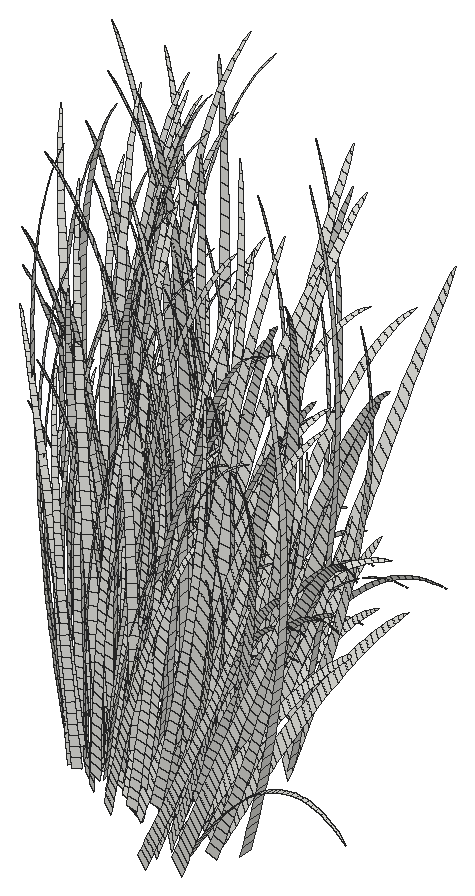
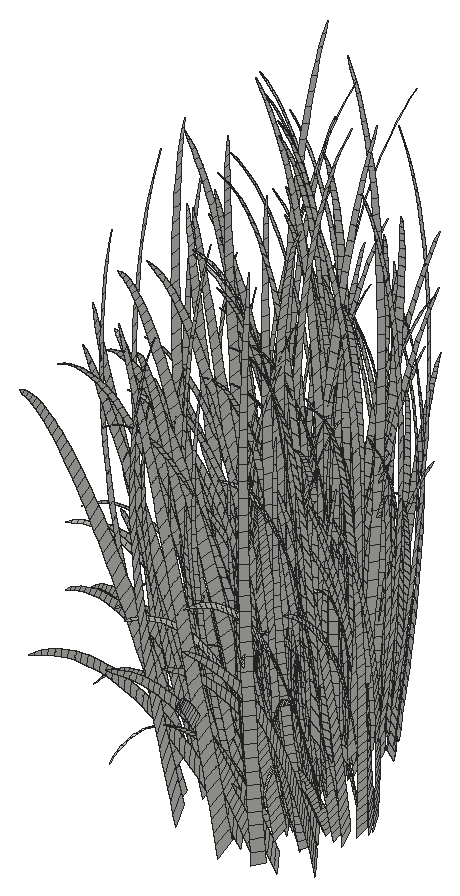
# SketchUp Ruby script. Lengths in inches.
U = 1.inch
M = Sketchup.active_model
def pt(a) = Geom::Point3d.new(a.map { |v| v * U })
def face(e, loops, mat)
  f = e.add_face(loops[0].map { |a| pt(a) })
  loops[1..].each { |l| e.add_face(l.map { |a| pt(a) }).erase! }
  f.material = f.back_material = mat if mat
  f
end
# faces: each face lists its corners as indices into pts; further lists are holes
def faces(e, pts, list, mat = nil) = list.each { |f| face(e, (f[0].is_a?(Array) ? f : [f]).map { |l| l.map { |i| pts[i] } }, mat) }
# xy, xz, yz: faces in a plane at the given z, y or x. An outline is a flat list of corners, or four numbers for a rectangle; further outlines are holes
def ring(l) = l.size == 4 ? [[l[0], l[1]], [l[2], l[1]], [l[2], l[3]], [l[0], l[3]]] : l.each_slice(2).to_a
def flat(e, list, mat, &to3) = list.each { |f| face(e, (f[0].is_a?(Array) ? f : [f]).map { |l| ring(l).map { |u, v| to3.(u, v) } }, mat) }
def xy(e, z, list, mat = nil) = flat(e, list, mat) { |x, y| [x, y, z] }
def xz(e, y, list, mat = nil) = flat(e, list, mat) { |x, z| [x, y, z] }
def yz(e, x, list, mat = nil) = flat(e, list, mat) { |y, z| [x, y, z] }
def lines(e, pts, list) = list.each { |a, b| e.add_line(pt(pts[a]), pt(pts[b])) }
# prism: a flat outline (further loops are holes) pulled along v
def prism(e, loops, v, mat = nil)
  f = face(e, loops, mat); d = Geom::Vector3d.new(v.map { |x| x * U })
  f.pushpull(f.normal.samedirection?(d) ? d.length : -d.length)
end
def box(e, o, s, mat = nil) = prism(e, [[o, [o[0] + s[0], o[1], o[2]], [o[0] + s[0], o[1] + s[1], o[2]], [o[0], o[1] + s[1], o[2]]]], [0, 0, s[2]], mat)
def at(x, y, z, deg = 0) = Geom::Transformation.translation(pt([x, y, z])) * Geom::Transformation.rotation(ORIGIN, Z_AXIS, deg.degrees)
def axes(o, x, y, z) = Geom::Transformation.new([*x, 0, *y, 0, *z, 0, *pt(o).to_a, 1])
def part(name) = M.definitions.add(name)
# library, detail: a bought-in or finely detailed component or shape, given as its bounding box
def library(name, o, s) = part(name).tap { |d| box(d.entities, o, s) }
def detail(e, o, s) = box(e.add_group.entities, o, s)
def put(e, d, t, mat = nil) = e.add_instance(d, t).tap { |i| i.material = mat if mat }
def group(e, t, mat = nil) = e.add_group.tap { |g| g.transformation = t; g.material = mat if mat }.entities
root = M.entities
c1 = part("fur_instance\#8")
p = [[-0.25,1.49,0.03],[0.25,-1.49,-0.03],[0.44,-1.47,1.51],[-0.05,1.47,1.57],[0.65,-1.44,3.05],[0.16,1.45,3.11],
  [0.86,-1.42,4.59],[0.38,1.44,4.65],[1.1,-1.39,6.13],[0.62,1.43,6.18],[1.34,-1.35,7.66],[0.875,1.42,7.72],
  [1.6,-1.32,9.19],[1.14,1.41,9.25],[1.88,-1.28,10.72],[1.43,1.41,10.78],[2.18,-1.24,12.25],[1.73,1.41,12.3],
  [2.49,-1.19,13.77],[2.05,1.41,13.82],[2.83,-1.15,15.29],[2.4,1.41,15.34],[3.18,-1.09,16.8],[2.76,1.42,16.85],
  [3.56,-1.03,18.31],[3.14,1.43,18.35],[3.96,-0.97,19.81],[3.55,1.44,19.85],[4.38,-0.91,21.3],[3.99,1.46,21.35],
  [4.84,-0.83,22.78],[4.45,1.48,22.83],[5.32,-0.76,24.26],[4.93,1.51,24.31],[5.82,-0.67,25.73],[5.45,1.54,25.77],
  [6.36,-0.59,27.18],[6,1.57,27.23],[6.93,-0.49,28.625],[6.58,1.61,28.67],[7.54,-0.39,30.05],[7.19,1.66,30.1],
  [8.18,-0.28,31.47],[7.84,1.71,31.51],[8.85,-0.16,32.86],[8.53,1.77,32.9],[9.57,-0.04,34.24],[9.25,1.83,34.27],
  [10.32,0.09,35.59],[10.02,1.9,35.625],[11.12,0.23,36.92],[10.82,1.97,36.95],[11.95,0.38,38.22],[11.67,2.06,38.25],
  [12.84,0.54,39.49],[12.57,2.14,39.52],[13.76,0.71,40.73],[13.51,2.24,40.76],[14.73,0.89,41.93],[14.49,2.34,41.95],
  [15.75,1.08,43.09],[15.52,2.45,43.11],[16.82,1.28,44.2],[16.6,2.5625,44.23],[17.93,1.5,45.27],[17.73,2.68,45.29],
  [19.08,1.73,46.28],[18.9,2.81,46.3],[20.29,1.97,47.24],[20.125,2.93,47.26],[21.53,2.22,48.13],[21.39,3.0625,48.15],
  [22.82,2.5,48.96],[22.7,3.1875,48.98],[24.14,2.8125,49.72],[24.06,3.3,49.73],[25.48,3.27,50.41]]
faces(c1.entities,p,[[0,1,2,3],[3,2,4,5],[5,4,6,7],[7,6,8,9],[9,8,10,11],[11,10,12,13],[13,12,14,15],[15,14,16,17],
  [17,16,18,19],[19,18,20,21],[21,20,22,23],[23,22,24,25],[25,24,26,27],[27,26,28,29],[29,28,30,31],[31,30,32,33],
  [33,32,34,35],[35,34,36,37],[37,36,38,39],[39,38,40,41],[41,40,42,43],[43,42,44,45],[45,44,46,47],[47,46,48,49],
  [49,48,50,51],[51,50,52,53],[53,52,54,55],[55,54,56,57],[57,56,58,59],[59,58,60,61],[61,60,62,63],[63,62,64,65],
  [65,64,66,67],[67,66,68,69],[69,68,70,71],[71,70,72,73],[73,72,74,75],[75,74,76]])
put(root,c1,axes([436.8,51.34,11.24],[0.12633,-0.01434,-0.33979],[0.03003,0.18353,-0.05493],[0.15045,-0.04633,0.28189]))
put(root,c1,axes([435.49,51.74,11.33],[-0.0586,-0.13145,0.25194],[0.10919,-0.10295,-0.16429],[0.12358,0.00811,0.25105]))
put(root,c1,axes([432.71,49.82,14.73],[-0.00201,0.1516,0.05729],[-0.16575,-0.0022,0.09935],[0.04109,-0.06021,0.3647]))
put(root,c1,axes([433.8,53.2,18.9],[-0.20879,-0.09834,0.1321],[0.10662,-0.20129,-0.08744],[0.06463,-0.06137,0.52082]))
put(root,c1,axes([436.89,53.59,13.54],[-0.04683,-0.20253,0.13494],[0.1704,-0.05617,-0.28372],[0.13472,-0.02969,0.38568]))
put(root,c1,axes([431.97,53.11,17.88],[0.1489,-0.1631,0.00196],[0.16131,0.12724,-0.0384],[0.00665,-0.0349,0.49014]))
put(root,c1,axes([431.66,49.77,14.8],[-0.04364,0.1509,0.04181],[-0.16335,-0.02313,-0.02043],[-0.0082,-0.05328,0.37608]))
put(root,c1,axes([433.46,51.77,15.9],[0.18544,-0.04972,-0.1199],[0.04511,0.1779,-0.04118],[0.05175,-0.03943,0.42412]))
put(root,c1,axes([433.6,49.6,13.46],[0.04868,0.13833,-0.04452],[-0.13249,0.04478,0.16098],[0.07098,-0.0404,0.31175]))
put(root,c1,axes([434.16,51.48,15.7],[0.19428,0.00099,-0.13011],[-0.00447,0.1857,0.01775],[0.05358,-0.05088,0.43173]))
put(root,c1,axes([430.26,50.87,15.53],[0.16328,0.03799,0.12354],[-0.06943,0.16853,-0.0179],[-0.05845,-0.04464,0.39911]))
put(root,c1,axes([439.11,52.69,11.72],[-0.15284,0.01805,0.42901],[-0.06641,-0.2167,0.01891],[0.18229,-0.0915,0.34824]))
put(root,c1,axes([431.49,50.18,15.65],[-0.11204,0.14362,0.03398],[-0.14775,-0.08605,-0.03808],[-0.00899,-0.05843,0.41243]))
put(root,c1,axes([429.22,52.28,18.31],[0.21896,0.00722,0.14738],[-0.05367,0.20894,0.06409],[-0.06377,-0.07981,0.49923]))
put(root,c1,axes([434.72,51.57,10.73],[-0.02967,-0.12807,0.22483],[0.11753,-0.07372,-0.14887],[0.10049,0.02798,0.22698]))
put(root,c1,axes([431.85,52.23,14.47],[-0.0829,-0.13844,0.09301],[0.15279,-0.09132,0.04718],[-0.00308,0.00854,0.37496]))
put(root,c1,axes([435.71,52.33,16.54],[-0.20296,0.04396,0.25147],[-0.06114,-0.20583,-0.00189],[0.10319,-0.08007,0.46398]))
put(root,c1,axes([431.41,50.68,14.82],[0.15712,0.04243,0.01115],[-0.06087,0.1538,-0.0283],[-0.01337,-0.02475,0.37716]))
put(root,c1,axes([435.26,50,11.07],[-0.0259,0.13847,0.08839],[-0.10293,-0.05886,0.26708],[0.12297,-0.03787,0.2304]))
put(root,c1,axes([436.86,50.52,11.18],[0.00679,0.17207,0.10989],[-0.13694,-0.04896,0.33579],[0.14998,-0.07528,0.28652]))
put(root,c1,axes([432.26,51.48,14.73],[0.16085,-0.07091,-0.00868],[0.05991,0.14859,-0.10356],[0.01607,0.00276,0.37166]))
put(root,c1,axes([432.51,51.87,13.23],[0.06075,-0.14439,0.11282],[0.14535,0.04045,-0.11615],[0.02704,0.02874,0.31908]))
put(root,c1,axes([430.1,50.88,15.83],[0.1306,0.09776,0.12408],[-0.13059,0.14634,-0.04229],[-0.05761,-0.05634,0.41276]))
put(root,c1,axes([430.4,52.76,15.81],[0.11915,-0.15444,0.11959],[0.14734,0.10329,0.01409],[-0.04397,-0.00116,0.41847]))
put(root,c1,axes([432.625,50.65,14.24],[0.15483,0.02452,-0.08835],[-0.03742,0.15266,-0.04583],[0.03016,-0.00858,0.34899]))
put(root,c1,axes([433.98,51.125,15.97],[-0.15292,0.11854,0.12624],[-0.12574,-0.14279,0.04956],[0.05301,-0.06232,0.4383]))
put(root,c1,axes([436.56,54.42,16.42],[0.1074,-0.20139,-0.09354],[0.19115,0.11076,-0.2385],[0.10824,-0.04151,0.48371]))
put(root,c1,axes([431.49,52.87,19.42],[0.24085,-0.01288,-0.01594],[-0.00713,0.21681,0.06326],[0.00207,-0.07616,0.53545]))
put(root,c1,axes([432.12,52.03,17.97],[0.21441,0.03504,-0.02755],[-0.05444,0.19871,0.04867],[0.01191,-0.06374,0.49276]))
put(root,c1,axes([432.125,50.6,14.6],[0.13491,0.07893,-0.02845],[-0.09527,0.13412,-0.00523],[0.005,-0.02625,0.36875]))
put(root,c1,axes([431.24,53.26,15.8125],[0.00836,-0.18662,0.11674],[0.19508,-0.00753,0.01588],[-0.01463,0.00988,0.4222]))
put(root,c1,axes([431.09,53.22,16.96],[-0.07053,-0.17965,0.10788],[0.19435,-0.08267,0.06265],[-0.01549,0.01046,0.44704]))
put(root,c1,axes([435.18,51.11,13.51],[-0.105,0.10997,0.20265],[-0.1047,-0.1341,0.17455],[0.11569,-0.04687,0.32514]))
put(root,c1,axes([432.1,52.89,15.32],[-0.10911,-0.1372,0.1051],[0.15387,-0.1168,0.04236],[0.00736,0.00708,0.40712]))
put(root,c1,axes([434.23,50.55,13.28],[-0.09933,0.11915,0.09682],[-0.11277,-0.10305,0.14649],[0.07419,-0.02845,0.33155]))
put(root,c1,axes([433.11,50.46,13.91],[0.12172,0.08749,-0.09823],[-0.09805,0.12464,0.01693],[0.03543,-0.01566,0.34464]))
put(root,c1,axes([430.63,50.98,15.98],[0.13112,0.1119,0.04642],[-0.13781,0.13647,-0.01148],[-0.02271,-0.04835,0.42618]))
put(root,c1,axes([430.55,51.83,16.41],[0.19137,0.02245,0.03812],[-0.04546,0.1843,-0.01629],[-0.02307,-0.03624,0.44138]))
put(root,c1,axes([434.53,52.1,14.78],[-0.17727,-0.00884,0.19718],[0.01815,-0.18643,0.05134],[0.08203,-0.01667,0.38902]))
put(root,c1,axes([433.12,52.07,18.65],[0.18476,0.1259,-0.03463],[-0.14125,0.16417,0.15823],[0.05053,-0.09421,0.50755]))
put(root,c1,axes([434.62,52.46,16.42],[-0.19467,0.01004,0.22404],[-0.00781,-0.20399,0.04036],[0.09618,-0.03688,0.42982]))
put(root,c1,axes([431.37,51.84,13.38],[-0.12985,-0.07677,0.07158],[0.09092,-0.12597,0.14453],[-0.01646,0.03757,0.31821]))
put(root,c1,axes([433.39,50.92,14.88],[0.10935,0.12723,-0.0806],[-0.13524,0.11022,0.08276],[0.04716,-0.03593,0.38648]))
put(root,c1,axes([429.38,54.24,20.375],[0.24246,-0.09581,0.04741],[0.07374,0.21618,0.03906],[-0.03158,-0.05994,0.56838]))
put(root,c1,axes([431.98,51.09,17.59],[-0.06667,0.19226,0.05915],[-0.20819,-0.04319,-0.00198],[0.00188,-0.06909,0.48578]))
put(root,c1,axes([434.43,50.96,14.39],[-0.05241,0.16147,0.07727],[-0.15892,-0.06034,0.18232],[0.08415,-0.0479,0.3696]))
put(root,c1,axes([433.22,52.97,13.9],[-0.09023,-0.13424,0.18354],[0.14991,-0.10591,-0.00994],[0.04513,0.02354,0.36032]))
put(root,c1,axes([432.84,53.1,13.82],[0.00974,-0.16765,0.16266],[0.17627,-0.01134,-0.08044],[0.03031,0.03221,0.35757]))
put(root,c1,axes([433.38,52.79,15.88],[0.18917,-0.06704,-0.06686],[0.05451,0.17895,-0.10326],[0.03727,-0.0106,0.43133]))
put(root,c1,axes([434.67,52.21,13.41],[0.15112,-0.07348,-0.15621],[0.04279,0.15836,-0.20373],[0.095,0.01621,0.32084]))
put(root,c1,axes([437.27,54.67,14.96],[0.12813,-0.17071,-0.17976],[0.14324,0.15198,-0.29056],[0.14651,-0.03228,0.41943]))
put(root,c1,axes([434.93,53.05,12.83],[0.12182,-0.13641,-0.05722],[0.10481,0.11532,-0.25636],[0.0972,0.01658,0.32827]))
put(root,c1,axes([435.92,53.18,13.58],[0.15027,-0.10781,-0.18095],[0.0791,0.16599,-0.22838],[0.11882,-0.00407,0.36105]))
put(root,c1,axes([430.77,53.96,15.66],[-0.05762,-0.17661,0.09378],[0.18885,-0.07013,0.07584],[-0.02585,0.00825,0.42914]))
put(root,c1,axes([435.62,53.42,12.85],[-0.08271,-0.14836,0.25336],[0.14839,-0.11682,-0.11362],[0.10275,0.01753,0.34702]))
put(root,c1,axes([434.1,51.39,13.31],[-0.15312,0.05179,0.12153],[-0.03636,-0.15379,0.12597],[0.06399,-0.0008,0.33763]))
put(root,c1,axes([433.56,53.75,17.9],[0.2045,-0.09371,-0.11076],[0.08595,0.19464,-0.09275],[0.05645,-0.03369,0.4916]))
put(root,c1,axes([432.29,52.34,16.85],[-0.20122,0.04978,0.02765],[-0.03696,-0.18587,0.02525],[0.00919,-0.0352,0.4569]))
put(root,c1,axes([430.86,50.42,14.45],[0.0007,0.15498,-0.03624],[-0.15701,0.01919,-0.0982],[-0.04789,-0.01409,0.35225]))
put(root,c1,axes([432.66,51.36,15.63],[0.15584,0.0797,-0.11547],[-0.0923,0.15744,0.00315],[0.04105,-0.01815,0.39937]))
put(root,c1,axes([429.87,52.42,15.4375],[0.18469,-0.02182,0.1026],[0.00322,0.18141,-0.06268],[-0.05045,-0.00814,0.41143]))
put(root,c1,axes([436.37,52.03,16.76],[0.03711,0.21617,0.09276],[-0.22705,0.0107,0.25479],[0.10293,-0.10542,0.49477]))
put(root,c1,axes([434.65,54.32,15.47],[-0.10531,-0.16415,0.20039],[0.16955,-0.12413,-0.09552],[0.08116,-0.00102,0.4282]))
put(root,c1,axes([431.16,50.85,14.77],[-0.005,0.15882,-0.01867],[-0.16818,0.01184,-0.02587],[-0.01594,-0.02637,0.37698]))
put(root,c1,axes([432.1,52.1,13.63],[-0.14817,-0.05096,0.10268],[0.07099,-0.14472,0.13123],[0.01339,0.03539,0.32926]))
put(root,c1,axes([431.96,51.06,14.67],[-0.14146,0.09732,-0.03277],[-0.08974,-0.12702,0.09515],[0.00654,0.00629,0.36155]))
put(root,c1,axes([431.49,53.55,20.54],[0.24462,0.04853,-0.00958],[-0.07419,0.22591,0.06737],[0.00661,-0.07917,0.56836]))
put(root,c1,axes([430.43,50.95,14.69],[0.07256,0.13813,0.01061],[-0.14853,0.08916,-0.10968],[-0.05042,-0.01484,0.37084]))
put(root,c1,axes([431.93,51.04,15.01],[0.0444,0.15353,-0.02873],[-0.16709,0.05572,0.00025],[-0.00083,-0.02443,0.38596]))
put(root,c1,axes([432.92,51.9,18.03],[0.00546,0.20018,0.07075],[-0.21886,0.00452,0.13393],[0.05427,-0.07952,0.48166]))
put(root,c1,axes([432.77,50.76,14.31],[0.01188,0.15545,-0.07184],[-0.16156,0.0237,0.07132],[0.03067,-0.00873,0.35494]))
put(root,c1,axes([432.97,53.13,17.9],[0.21551,0.00607,-0.13742],[-0.0172,0.21045,-0.03067],[0.05502,-0.03283,0.47913]))
put(root,c1,axes([431.2,53.64,16.84],[0.17834,-0.11625,0.08266],[0.1071,0.16149,-0.09447],[-0.01558,0.01053,0.44981]))
put(root,c1,axes([431.7,51.0625,14.4375],[-0.12044,0.11617,-0.06507],[-0.11184,-0.10532,0.07409],[-0.00291,0.00808,0.35453]))
put(root,c1,axes([432.59,54.67,16.55],[-0.12335,-0.15584,0.12717],[0.17408,-0.13265,0.02266],[0.01997,0.00343,0.46197]))
put(root,c1,axes([432.86,51.29,13.95],[-0.11227,0.12169,-0.01571],[-0.11695,-0.0983,0.09825],[0.0234,-0.00238,0.35291]))
put(root,c1,axes([436.11,52.24,15.86],[-0.05009,0.1972,0.12811],[-0.20341,-0.06615,0.21296],[0.10198,-0.07913,0.45854]))
put(root,c1,axes([432.14,52.43,13.0625],[-0.15178,-0.03817,0.09021],[0.05761,-0.14672,0.13772],[0.01323,0.03497,0.32535]))
put(root,c1,axes([432.78,56.22,20.72],[-0.01557,-0.2472,0.11257],[0.25666,-0.03446,-0.11464],[0.04868,-0.01385,0.56337]))
put(root,c1,axes([432.09,51.68,17.12],[0.00321,0.19067,0.02092],[-0.20749,0.01649,0.04397],[0.01444,-0.0534,0.46311]))
put(root,c1,axes([437.05,56.51,16.92],[0.03522,-0.24577,0.05534],[0.23308,0.0235,-0.26379],[0.10852,-0.02206,0.51462]))
put(root,c1,axes([433.91,51.8,12.53],[0.1392,0.01865,-0.19659],[-0.04604,0.15192,-0.11441],[0.07206,0.03039,0.28637]))
put(root,c1,axes([432.01,52.86,20.18],[0.1638,0.16225,0.02835],[-0.19372,0.16204,0.06129],[0.00656,-0.07857,0.56406]))
put(root,c1,axes([435.66,52.24,15.02],[0.10459,0.17012,-0.10766],[-0.16118,0.10117,0.20027],[0.09662,-0.055,0.42437]))
put(root,c1,axes([430.55,52.39,14.6],[0.167,0.03821,0.03014],[-0.05354,0.16593,-0.1048],[-0.03226,0.00399,0.38398]))
put(root,c1,axes([430.77,52.4,18.79],[-0.07149,0.20688,0.05021],[-0.22153,-0.04139,-0.03916],[-0.01557,-0.07173,0.51835]))
put(root,c1,axes([435.7,51.74,13.15],[-0.05226,0.17384,0.04608],[-0.14605,-0.06174,0.27189],[0.11826,-0.02606,0.33853]))
put(root,c1,axes([431.3,52.43,14.34],[0.17226,-0.02677,0.04434],[0.01787,0.15893,-0.17055],[-0.01798,0.04104,0.34767]))
put(root,c1,axes([431.4375,55.84,18.58],[-0.01914,-0.22341,0.14227],[0.23668,-0.03758,0.00754],[-0.0042,0.01167,0.5122]))
put(root,c1,axes([434.17,51.02,12.7],[-0.0035,0.15221,-0.13037],[-0.13811,0.0204,0.18439],[0.08356,0.01425,0.28222]))
put(root,c1,axes([428.65,53.91,17.6875],[0.21533,-0.00022,0.14201],[-0.02985,0.21622,-0.04212],[-0.07083,-0.0307,0.48991]))
put(root,c1,axes([437.2,52.61,10.97],[-0.11534,0.10838,0.24896],[-0.07338,-0.1624,0.25205],[0.15325,-0.01897,0.29298]))
put(root,c1,axes([433.06,52.68,12.9],[0.15705,-0.06817,-0.01855],[0.04537,0.13415,-0.23216],[0.04015,0.05663,0.29621]))
put(root,c1,axes([434.03,55.28,17.3],[0.13505,-0.18869,0.02697],[0.17317,0.11473,-0.23558],[0.07413,0.01575,0.4615]))
put(root,c1,axes([432.33,52.5625,19.45],[-0.01737,0.2214,0.05487],[-0.24332,0.00145,0.03189],[0.01003,-0.07326,0.54284]))
put(root,c1,axes([432.12,51.49,14.94],[0.04623,0.15623,-0.10375],[-0.16763,0.05842,0.01792],[0.01628,0.0028,0.37652]))
put(root,c1,axes([431.4,54.43,14.33],[0.1059,-0.15637,0.15831],[0.16025,0.08485,-0.11228],[-0.00207,0.04487,0.3837]))
put(root,c1,axes([436.29,53.27,16.98],[-0.13857,0.17143,0.18015],[-0.17196,-0.14956,0.18932],[0.11106,-0.06322,0.48777]))
put(root,c1,axes([432.57,52.36,17.125],[-0.03706,0.19452,0.0025],[-0.2058,-0.02021,0.04233],[0.01369,-0.04269,0.4672]))
put(root,c1,axes([431.26,54.78,14.45],[0.06236,-0.17527,0.19539],[0.18475,0.04701,-0.03446],[-0.02024,0.04621,0.39144]))
put(root,c1,axes([430.72,54.83,14.47],[0.05449,-0.17808,0.19773],[0.18828,0.03949,-0.026],[-0.02035,0.04645,0.39347]))
put(root,c1,axes([432.55,52.26,12.76],[-0.15815,0.00988,0.0597],[0.01239,-0.13945,0.21255],[0.01922,0.06125,0.28145]))
put(root,c1,axes([432.38,52.875,19.76],[0.06704,0.21243,0.03183],[-0.23851,0.07708,0.05394],[0.01333,-0.07138,0.55186]))
put(root,c1,axes([434.53,55.86,19.01],[-0.21942,-0.09635,0.15751],[0.11362,-0.22061,0.00466],[0.05601,-0.02476,0.54483]))
put(root,c1,axes([432.95,52.63,18.42],[0.01128,0.21113,0.01155],[-0.2291,0.02553,0.05014],[0.01651,-0.05502,0.51224]))
put(root,c1,axes([434.15,53.9,10.9],[-0.03747,-0.12843,0.29203],[0.15407,-0.08219,-0.0652],[0.07562,0.07004,0.25518]))
put(root,c1,axes([431.83,53.28,20.15],[0.09204,0.20501,0.03679],[-0.23374,0.09978,0.05402],[0.01033,-0.07544,0.55902]))
put(root,c1,axes([433.64,52.66,16.98],[0.05117,0.19348,-0.04619],[-0.20175,0.05612,0.13032],[0.05644,-0.043,0.46253]))
put(root,c1,axes([430.41,52.48,13.43],[0.14782,0.0607,0.01728],[-0.06736,0.14608,-0.17165],[-0.04658,0.03213,0.33667]))
put(root,c1,axes([433,51.77,12.82],[-0.04536,0.14528,-0.12173],[-0.14819,-0.02558,0.10276],[0.0266,0.02828,0.3139]))
put(root,c1,axes([431.81,53.54,14.71],[0.18587,-0.039,0.02017],[0.0261,0.16941,-0.18858],[-0.00202,0.04384,0.37494]))
put(root,c1,axes([430.6,55.93,20.69],[0.25389,-0.06297,0.01758],[0.0429,0.23535,-0.03956],[-0.01113,-0.0353,0.57531]))
put(root,c1,axes([432.52,53.94,17.13],[-0.20845,0.0617,0.05447],[-0.04632,-0.1966,0.1192],[0.03082,-0.00313,0.46484]))
put(root,c1,axes([429.74,54.01,12.15],[0.12753,-0.09379,0.22491],[0.10527,0.1265,-0.10063],[-0.06372,0.06207,0.3109]))
put(root,c1,axes([430.05,52.88,11.86],[0.15191,0.00864,0.09894],[-0.00116,0.14441,-0.20359],[-0.05853,0.05702,0.28561]))
put(root,c1,axes([435.86,52.16,11.28],[0.00579,0.17068,-0.16321],[-0.12957,0.03754,0.26919],[0.12935,0.00849,0.26276]))
put(root,c1,axes([429.66,53.07,12.26],[0.15072,0.0136,0.13727],[-0.00409,0.15385,-0.193],[-0.07769,0.04892,0.29677]))
put(root,c1,axes([431.37,53.83,11.47],[-0.01699,-0.12732,0.27857],[0.16448,-0.01291,0.05595],[-0.02464,0.09551,0.24356]))
put(root,c1,axes([429.25,55.34,17.07],[0.21265,-0.06804,0.11906],[0.05038,0.20319,-0.07151],[-0.05071,-0.00134,0.48262]))
put(root,c1,axes([434.58,53.23,13.37],[-0.16864,0.05731,0.14747],[-0.02228,-0.16808,0.21885],[0.0836,0.03526,0.33224]))
put(root,c1,axes([434.18,54.21,11.59],[0.14782,-0.11273,0.00048],[0.0732,0.11159,-0.31128],[0.07867,0.07287,0.26546]))
put(root,c1,axes([432.83,54.28,11.07],[0.01055,-0.13508,0.28615],[0.17058,-0.02073,-0.06684],[0.02674,0.09288,0.2522]))
put(root,c1,axes([434.67,53.03,15.79],[0.08157,0.17825,-0.15725],[-0.17491,0.09532,0.15482],[0.08885,-0.01806,0.42132]))
put(root,c1,axes([430.125,53.37,12.92],[0.16194,-0.0082,0.12991],[0.01706,0.15486,-0.20493],[-0.06274,0.06113,0.30616]))
put(root,c1,axes([431.16,52.18,13.79],[0.03769,0.14922,-0.14278],[-0.15939,0.04231,-0.09138],[-0.03216,0.03689,0.33298]))
put(root,c1,axes([431.29,52.41,12.53],[0.13054,0.07134,-0.09742],[-0.08675,0.11604,-0.1956],[-0.0202,0.06504,0.27821]))
put(root,c1,axes([433.83,55.2,12.58],[-0.10724,-0.12303,0.26265],[0.15657,-0.12402,0.06415],[0.04661,0.06574,0.34387]))
put(root,c1,axes([432.77,53.06,11.25],[-0.15615,0.01011,0.08042],[0.021,-0.12557,0.25868],[0.02465,0.08562,0.2325]))
put(root,c1,axes([432.77,53.58,15.1],[-0.18299,0.07424,0.021],[-0.05602,-0.16634,0.19558],[0.03285,0.03492,0.38761]))
put(root,c1,axes([430.76,53.42,18.14],[-0.02533,0.21082,-0.03246],[-0.22123,-0.00286,-0.02372],[-0.01766,-0.03271,0.49841]))
put(root,c1,axes([432.92,55.3125,19.96],[-0.23935,0.06874,0.11641],[-0.05487,-0.22915,0.10476],[0.05566,-0.0246,0.54145]))
put(root,c1,axes([431.97,52.94,15.625],[-0.04271,0.18174,-0.10347],[-0.18723,-0.02484,0.051],[0.00749,0.00721,0.41447]))
put(root,c1,axes([435.88,53.53,11.66],[-0.14434,0.09377,0.17872],[-0.03919,-0.15638,0.28066],[0.124,0.03453,0.28007]))
put(root,c1,axes([435.47,53.59,14.2],[0.1044,0.14559,-0.25751],[-0.13502,0.13555,0.13946],[0.11942,-0.00409,0.36287]))
put(root,c1,axes([435.07,53.65,17.56],[0.01228,0.22259,-0.04839],[-0.21245,0.01489,0.2439],[0.10506,-0.04029,0.46949]))
put(root,c1,axes([430.93,54.26,11.63],[0.1046,-0.10479,0.24905],[0.1356,0.08115,-0.15676],[-0.02552,0.09892,0.25225]))
put(root,c1,axes([434.4,53.625,13.03],[-0.15929,0.09132,0.09708],[-0.05737,-0.15132,0.24406],[0.08321,0.03509,0.33068]))
put(root,c1,axes([433.91,53.21,11.63],[-0.15229,0.06835,0.08842],[-0.02287,-0.13137,0.27682],[0.07344,0.06802,0.24782]))
put(root,c1,axes([434.22,52.82,11.76],[-0.11038,0.13094,-0.01587],[-0.09023,-0.08182,0.28993],[0.09271,0.05046,0.24619]))
put(root,c1,axes([432.73,53.39,12.67],[0.1552,0.04284,-0.14088],[-0.07244,0.14474,-0.19228],[0.02075,0.06614,0.30388]))
put(root,c1,axes([430.6875,54.09,16.92],[0.1688,0.10784,-0.0329],[-0.12628,0.17185,-0.12449],[-0.0276,0.0088,0.45819]))
put(root,c1,axes([436.36,53.58,11.05],[-0.08133,0.16944,0.041],[-0.11353,-0.08181,0.33645],[0.13926,0.00914,0.28291]))
put(root,c1,axes([433.3125,55.02,16.03],[0.2064,0.00506,-0.149],[-0.0314,0.20396,-0.16093],[0.05385,0.02809,0.42994]))
put(root,c1,axes([433.39,53.49,13.66],[-0.1523,0.1081,0.01181],[-0.08113,-0.12936,0.25496],[0.06382,0.04964,0.32324]))
put(root,c1,axes([430.04,54.79,12.04],[0.16515,-0.05448,0.15409],[0.06343,0.14946,-0.20076],[-0.0453,0.07156,0.32105]))
put(root,c1,axes([433.1,55.9,14.4],[0.16589,-0.13509,0.0734],[0.11769,0.12965,-0.28034],[0.04996,0.07046,0.36857]))
put(root,c1,axes([435.36,54.95,13.29],[0.18376,0.00291,-0.23488],[-0.03958,0.19621,-0.17283],[0.09238,0.03896,0.36714]))
put(root,c1,axes([434.46,55.05,12.71],[0.18658,-0.03164,-0.14855],[-0.00603,0.17961,-0.23275],[0.06904,0.0537,0.34969]))
put(root,c1,axes([435.53,55.53,11.7],[-0.14001,-0.05504,0.33454],[0.10116,-0.17879,0.10883],[0.11232,0.06113,0.29828]))
put(root,c1,axes([438.43,56.86,14.06],[-0.20751,-0.0154,0.34807],[0.03231,-0.24429,0.09326],[0.14695,-0.00503,0.44651]))
put(root,c1,axes([431.7,57.52,16.6],[0.08686,-0.20683,0.21585],[0.21659,0.06277,-0.09493],[-0.00252,0.05451,0.46618]))
put(root,c1,axes([432.53,55.2,14.41],[-0.20063,0.02155,0.04243],[-0.00141,-0.18611,0.19899],[0.01635,0.04322,0.40207]))
put(root,c1,axes([437.375,57.76,13.18],[-0.06693,-0.18459,0.37403],[0.17622,-0.13687,-0.1896],[0.15627,0.04352,0.35297]))
put(root,c1,axes([431.97,55.79,13.99],[0.16091,-0.11894,0.16216],[0.12315,0.12828,-0.22813],[-0.0007,0.08282,0.35694]))
put(root,c1,axes([436.61,53.85,11.18],[-0.00334,0.19157,-0.16025],[-0.14373,0.02868,0.30995],[0.14337,0.00941,0.29124]))
put(root,c1,axes([433.76,55.45,15.32],[-0.20765,0.04551,0.10452],[-0.02061,-0.19877,0.19268],[0.05382,0.02807,0.42972]))
put(root,c1,axes([435.69,57.97,14.13],[0.12626,-0.20284,0.07113],[0.17291,0.09387,-0.32445],[0.10522,0.04438,0.41818]))
put(root,c1,axes([433.32,53.3,12.58],[0.03504,0.14333,-0.23786],[-0.16522,0.06024,0.03644],[0.04149,0.05851,0.30605]))
put(root,c1,axes([430.05,53.64,12.9],[0.12802,0.10582,-0.05497],[-0.1046,0.11656,-0.24012],[-0.0637,0.06206,0.31081]))
put(root,c1,axes([433.45,54.25,13.22],[-0.17132,0.08809,0.00001],[-0.06467,-0.14373,0.26091],[0.04498,0.06344,0.33183]))
put(root,c1,axes([433.51,54.82,11.52],[-0.16842,0.00001,0.17613],[0.0504,-0.15213,0.25899],[0.055,0.08838,0.2682]))
put(root,c1,axes([432.14,53.36,11.07],[-0.06121,0.11818,-0.24749],[-0.14799,-0.03414,0.11286],[0.00064,0.09094,0.23354]))
put(root,c1,axes([429.92,54.43,17.15],[0.03814,0.2015,-0.09604],[-0.21147,0.05412,-0.09289],[-0.03952,0.00488,0.47049]))
put(root,c1,axes([431.15,56.53,11.93],[0.03807,-0.14827,0.33406],[0.19165,0.02974,-0.03379],[-0.02912,0.11286,0.28781]))
put(root,c1,axes([435.17,56.89,11.44],[-0.12598,-0.09298,0.35138],[0.14548,-0.16001,0.09177],[0.09178,0.08501,0.30971]))
put(root,c1,axes([434.57,58.12,14.43],[0.17475,-0.1628,0.03799],[0.13362,0.1403,-0.32315],[0.08136,0.06328,0.41208]))
put(root,c1,axes([433.52,57.27,11.34],[-0.04728,-0.14736,0.35137],[0.1919,-0.08682,-0.02284],[0.06183,0.09936,0.30152]))
put(root,c1,axes([434.77,58.26,13.875],[-0.12567,-0.14648,0.32324],[0.17955,-0.15616,0.02426],[0.08105,0.06304,0.41053]))
put(root,c1,axes([435.65,54.58,12.23],[-0.05675,0.18901,-0.12396],[-0.14509,-0.01855,0.32364],[0.12915,0.03597,0.29172]))
put(root,c1,axes([432.7,56.13,19.51],[-0.19584,0.16179,-0.00169],[-0.1515,-0.17581,0.15196],[0.03573,-0.00363,0.539]))
put(root,c1,axes([432.45,55.25,17.15],[0.03623,0.20627,-0.12936],[-0.21911,0.05324,0.03667],[0.02079,0.00357,0.48088]))
put(root,c1,axes([431.47,55.09,11.91],[0.17646,0.02205,-0.09309],[-0.04854,0.13883,-0.29657],[0.00073,0.10392,0.26687]))
put(root,c1,axes([431.35,56.29,20.87],[0.11288,0.21144,-0.04258],[-0.23471,0.1258,-0.00774],[-0.00125,-0.03681,0.58142]))
put(root,c1,axes([435.2,54.68,11.28],[-0.02741,0.17392,-0.23076],[-0.16029,0.02766,0.23757],[0.10574,0.05755,0.28081]))
put(root,c1,axes([435.95,56.28,16.52],[0.06433,0.21786,-0.19116],[-0.21809,0.08663,0.16557],[0.09246,-0.00116,0.48782]))
put(root,c1,axes([435.55,57.17,12.19],[-0.18323,0.03397,0.2678],[0.02904,-0.19802,0.26654],[0.12063,0.06566,0.32036]))
put(root,c1,axes([432.27,56.03,14.99],[-0.1319,0.16634,-0.13442],[-0.16484,-0.10583,0.16664],[0.0172,0.04548,0.42308]))
put(root,c1,axes([432.2,56.15,12.69],[0.16157,0.07757,-0.19831],[-0.11325,0.15562,-0.18994],[0.0239,0.07619,0.35007]))
put(root,c1,axes([431.82,55.72,11.7],[-0.17438,0.07052,-0.11324],[-0.07295,-0.12692,0.30042],[0.00076,0.10733,0.27565]))
put(root,c1,axes([433.63,56.33,17.2],[0.08086,0.19655,-0.23287],[-0.213,0.10459,0.05528],[0.05877,0.03065,0.4692]))
put(root,c1,axes([432.5,58.73,13.55],[-0.18748,-0.08453,0.22152],[0.12512,-0.17975,0.22209],[0.0273,0.08703,0.39989]))
put(root,c1,axes([433.93,55.47,11.65],[0.02265,0.14627,-0.32338],[-0.18321,0.06424,0.06],[0.05776,0.09281,0.28164]))
put(root,c1,axes([434.89,56.84,18.81],[-0.06671,0.24175,-0.07521],[-0.22931,-0.04686,0.25475],[0.09711,-0.00122,0.51237]))
put(root,c1,axes([430.61,56.1,14.49],[0.14274,0.1248,-0.18106],[-0.14873,0.12853,-0.2232],[-0.02656,0.08555,0.36591]))
put(root,c1,axes([429.72,56.78,15.77],[0.14854,0.14611,-0.10639],[-0.16099,0.14725,-0.20019],[-0.04301,0.04934,0.44533]))
put(root,c1,axes([429.82,57.37,18.55],[0.10044,0.20522,-0.10286],[-0.22219,0.11383,-0.10772],[-0.03192,0.01018,0.52996]))
put(root,c1,axes([429.98,58.02,19.98],[0.19334,0.14897,-0.05271],[-0.17118,0.19893,-0.14866],[-0.0338,0.01079,0.56126]))
put(root,c1,axes([435.11,57.3,16.53],[-0.1067,0.21804,-0.07354],[-0.20586,-0.08261,0.23931],[0.07827,0.01663,0.48727]))
put(root,c1,axes([432.12,57.33,11.15],[0.19789,0.01674,-0.08664],[-0.04397,0.1548,-0.33323],[0.00081,0.11511,0.29561]))
put(root,c1,axes([433.9,57.8,12.05],[0.19779,0.00085,-0.20861],[-0.06023,0.17892,-0.30359],[0.06469,0.10395,0.31543]))
put(root,c1,axes([434.18,57.3,18.32],[-0.0236,0.24008,-0.16159],[-0.23761,0.00409,0.20091],[0.0806,0.01712,0.5018]))
put(root,c1,axes([431.94,57.36,12.73],[-0.13558,0.14856,-0.21429],[-0.16001,-0.10351,0.19496],[-0.00072,0.08572,0.36945]))
put(root,c1,axes([429.4,57.84,12.28],[0.1975,0.05806,-0.0072],[-0.05058,0.15655,-0.36297],[-0.06266,0.11673,0.31011]))
put(root,c1,axes([436.89,58.56,15.6],[-0.08095,0.24089,-0.09572],[-0.20653,-0.05261,0.34972],[0.13417,0.02289,0.45313]))
put(root,c1,axes([429.3,62.27,14.23],[0.05792,-0.21665,0.35228],[0.2474,0.04272,-0.03732],[-0.03274,0.10545,0.45101]))
put(root,c1,axes([431.82,61.65,13.85],[0.18259,-0.1619,0.22728],[0.17109,0.14301,-0.26039],[-0.00086,0.10227,0.44077]))
put(root,c1,axes([435.47,60.48,13.87],[-0.23752,0.04727,0.17981],[0.00037,-0.22718,0.3018],[0.08784,0.06833,0.44492]))
put(root,c1,axes([432.77,58.19,12.5],[-0.15443,0.14355,-0.21021],[-0.15015,-0.09516,0.30489],[0.0337,0.11705,0.31784]))
